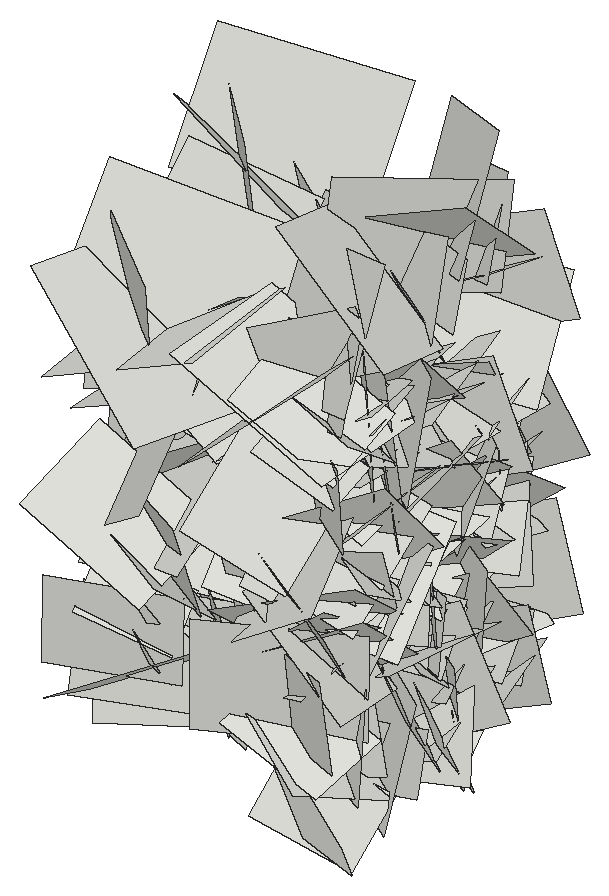
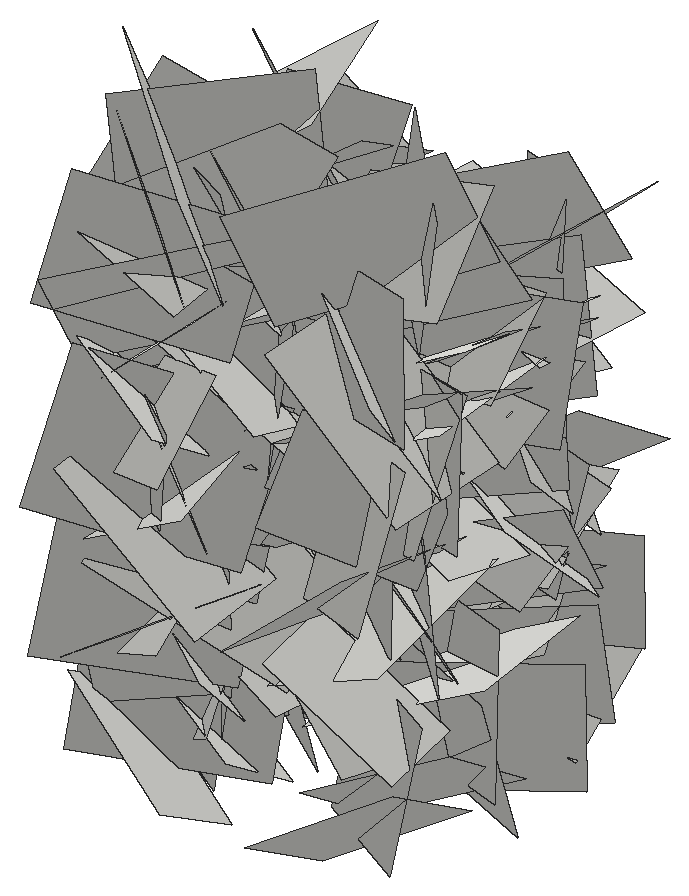
# SketchUp Ruby script. Lengths in inches.
U = 1.inch
M = Sketchup.active_model
def pt(a) = Geom::Point3d.new(a.map { |v| v * U })
def face(e, loops, mat)
  f = e.add_face(loops[0].map { |a| pt(a) })
  loops[1..].each { |l| e.add_face(l.map { |a| pt(a) }).erase! }
  f.material = f.back_material = mat if mat
  f
end
# faces: each face lists its corners as indices into pts; further lists are holes
def faces(e, pts, list, mat = nil) = list.each { |f| face(e, (f[0].is_a?(Array) ? f : [f]).map { |l| l.map { |i| pts[i] } }, mat) }
# xy, xz, yz: faces in a plane at the given z, y or x. An outline is a flat list of corners, or four numbers for a rectangle; further outlines are holes
def ring(l) = l.size == 4 ? [[l[0], l[1]], [l[2], l[1]], [l[2], l[3]], [l[0], l[3]]] : l.each_slice(2).to_a
def flat(e, list, mat, &to3) = list.each { |f| face(e, (f[0].is_a?(Array) ? f : [f]).map { |l| ring(l).map { |u, v| to3.(u, v) } }, mat) }
def xy(e, z, list, mat = nil) = flat(e, list, mat) { |x, y| [x, y, z] }
def xz(e, y, list, mat = nil) = flat(e, list, mat) { |x, z| [x, y, z] }
def yz(e, x, list, mat = nil) = flat(e, list, mat) { |y, z| [x, y, z] }
def lines(e, pts, list) = list.each { |a, b| e.add_line(pt(pts[a]), pt(pts[b])) }
# prism: a flat outline (further loops are holes) pulled along v
def prism(e, loops, v, mat = nil)
  f = face(e, loops, mat); d = Geom::Vector3d.new(v.map { |x| x * U })
  f.pushpull(f.normal.samedirection?(d) ? d.length : -d.length)
end
def box(e, o, s, mat = nil) = prism(e, [[o, [o[0] + s[0], o[1], o[2]], [o[0] + s[0], o[1] + s[1], o[2]], [o[0], o[1] + s[1], o[2]]]], [0, 0, s[2]], mat)
def at(x, y, z, deg = 0) = Geom::Transformation.translation(pt([x, y, z])) * Geom::Transformation.rotation(ORIGIN, Z_AXIS, deg.degrees)
def axes(o, x, y, z) = Geom::Transformation.new([*x, 0, *y, 0, *z, 0, *pt(o).to_a, 1])
def part(name) = M.definitions.add(name)
# library, detail: a bought-in or finely detailed component or shape, given as its bounding box
def library(name, o, s) = part(name).tap { |d| box(d.entities, o, s) }
def detail(e, o, s) = box(e.add_group.entities, o, s)
def put(e, d, t, mat = nil) = e.add_instance(d, t).tap { |i| i.material = mat if mat }
def group(e, t, mat = nil) = e.add_group.tap { |g| g.transformation = t; g.material = mat if mat }.entities
root = M.entities
c1 = part("Component\#6")
p = [[0.01,0,0],[0,3.24,4.54],[4.32,3.24,4.54],[4.33,0,0]]
faces(c1.entities,p,[[0,1,2,3]])
put(root,c1,axes([14.53,158.45,22.43],[-0.19892,0.24365,-1.12098],[0.08242,-1.13056,-0.25875],[1.21318,0.11676,-0.16622]))
put(root,c1,axes([14.53,153.47,7.93],[-0.25077,0.36385,-1.26635],[-0.08689,-1.28818,-0.35481],[1.39394,-0.01484,-0.24993]))
put(root,c1,axes([18.5,151.91,13.09],[0.06029,-0.61389,0.14039],[-0.0496,0.13645,0.61563],[-0.66568,-0.06576,-0.03315]))
put(root,c1,axes([18.5,155.37,8.05],[0.03179,-0.04018,0.69029],[0.07893,0.6871,0.03676],[-0.72868,0.07267,0.03409]))
put(root,c1,axes([18.5,147.25,18.09],[0.11506,-0.20062,0.68841],[0.02156,0.69683,0.19986],[-0.75976,-0.01061,0.10993]))
put(root,c1,axes([18.5,146,16.15],[0.10062,0.63244,0.10884],[-0.07256,0.11937,-0.63396],[-0.67636,0.08128,0.0842]))
put(root,c1,axes([14.53,157.74,11.21],[0.0595,-0.6331,0.72554],[0.06262,0.72766,0.63038],[1.01877,-0.00775,-0.08112]))
put(root,c1,axes([14.53,160.22,19.0625],[-0.13961,-0.68099,-1.03193],[-0.07146,-1.03227,0.68982],[1.30861,-0.12902,-0.07242]))
put(root,c1,axes([18.5,149.02,5.32],[0.19432,-0.67994,0.40742],[0.04988,0.42677,0.69106],[-0.83874,-0.13215,0.13549]))
put(root,c1,axes([14.53,154.9,1.8],[0.03269,0.90387,0.50014],[0.00572,0.50021,-0.90434],[1.09498,-0.0296,-0.01021]))
put(root,c1,axes([18.5,152.72,13.34],[0.14332,-0.62648,-0.12325],[-0.10799,-0.14554,0.62801],[-0.66813,-0.11086,-0.12794]))
put(root,c1,axes([14.53,157.43,12.97],[-0.1074,-0.05602,-1.35571],[-0.22854,-1.34155,0.07155],[1.42001,-0.22014,-0.09102]))
put(root,c1,axes([14.53,151.01,19.39],[0.01021,0.65154,-0.69294],[0.23408,-0.67557,-0.63214],[0.98066,0.15447,0.1581]))
put(root,c1,axes([14.53,148.31,17.26],[0.09379,0.98835,0.28145],[-0.01751,0.28383,-0.99149],[1.08916,-0.08054,-0.04018]))
put(root,c1,axes([14.53,155.4,17.52],[-0.19723,0.3027,-1.19403],[0.0763,-1.20284,-0.31615],[1.30348,0.11621,-0.16216]))
put(root,c1,axes([14.53,145.87,3.84],[0.08046,-0.07863,0.91675],[0.19442,0.90269,0.06223],[0.95574,-0.17701,-0.08983]))
put(root,c1,axes([14.53,148.09,7.11],[-0.15706,0.67864,1.02073],[0.03183,1.02986,-0.68036],[1.29889,0.05683,0.1401]))
put(root,c1,axes([14.53,148.93,-0.125],[-0.17085,0.2332,1.25619],[-0.02467,1.2654,-0.2379],[1.35409,0.05247,0.15416]))
put(root,c1,axes([14.53,158.83,13.98],[0.00743,-1.2386,0.03478],[-0.17851,0.0335,1.22715],[1.30124,0.01167,0.16814]))
put(root,c1,axes([14.53,152.08,1.74],[0.04493,0.85391,0.54577],[0.09586,0.54089,-0.85328],[1.06994,-0.08432,0.05353]))
put(root,c1,axes([14.53,151.75,19.45],[0.16935,0.44212,0.83371],[0.05466,0.84022,-0.45546],[0.99881,-0.12095,-0.11643]))
put(root,c1,axes([18.5,150.18,6.375],[0.17639,-0.58204,-0.33942],[-0.00316,-0.35025,0.59915],[-0.71419,-0.1422,-0.08648]))
put(root,c1,axes([18.5,148.65,3.04],[0.12439,-0.47488,0.46679],[0.05284,0.47892,0.47469],[-0.70386,-0.04797,0.11813]))
put(root,c1,axes([14.53,156.6875,24.44],[0.16473,0.01802,-1.18121],[-0.23771,-1.16927,-0.04735],[1.22945,-0.22849,0.14911]))
put(root,c1,axes([14.53,147.43,1.76],[0.0449,0.15818,1.07958],[0.0304,1.07985,-0.15935],[1.15617,-0.03454,-0.03773]))
put(root,c1,axes([14.53,158.38,15.93],[-0.03304,0.59909,-1.16183],[-0.1621,-1.15585,-0.5919],[1.37611,-0.12177,-0.09762]))
put(root,c1,axes([14.53,156.09,10.89],[0.02844,-1.01096,-0.23497],[0.17327,-0.228,0.99963],[1.08645,0.06282,-0.15327]))
put(root,c1,axes([14.53,159.05,4.5],[0.22831,-0.97739,-0.02602],[-0.01319,-0.02938,1.00067],[1.03632,0.21495,0.01847]))
put(root,c1,axes([14.53,157.5,5.99],[0.02733,0.34478,-1.12821],[-0.04378,-1.12752,-0.34552],[1.24973,-0.04704,0.01257]))
put(root,c1,axes([14.53,147.25,11.15],[0.01251,0.83252,-0.66438],[0.16644,-0.65852,-0.82239],[1.1167,0.08883,0.13002]))
put(root,c1,axes([18.5,155.94,6.59],[0.14653,0.65267,0.04592],[0.0729,0.03218,-0.6644],[-0.6897,0.14207,-0.06047]))
put(root,c1,axes([14.53,153.16,13.74],[0.07693,-1.07175,0.44962],[-0.07215,0.4458,1.07364],[1.22986,0.09319,0.03486]))
put(root,c1,axes([14.53,150.33,13.2],[-0.24126,0.02501,1.36725],[0.05252,1.3853,-0.01709],[1.44858,-0.04606,0.22834]))
put(root,c1,axes([14.53,144.59,11.1],[0.20686,0.83944,0.54314],[0.00436,0.55271,-0.85571],[1.05982,-0.16612,-0.10249]))
put(root,c1,axes([14.53,153.72,24.55],[-0.10736,0.8301,-0.78481],[0.26067,-0.75358,-0.8288],[1.18252,0.24148,0.11144]))
put(root,c1,axes([14.53,148.8125,12.02],[0.02959,0.36254,-1.01381],[0.21176,-0.99828,-0.35148],[1.12146,0.17893,0.09312]))
put(root,c1,axes([14.53,148.37,14.37],[0.13394,0.02599,1.3483],[-0.3112,1.32226,0.00203],[1.39518,0.29244,-0.12899]))
put(root,c1,axes([14.53,151.84,12.71],[0.09641,-0.969,-0.91768],[-0.24854,-0.9171,0.94515],[1.39265,-0.09659,0.2322]))
put(root,c1,axes([14.53,152.41,8.09],[-0.02535,-1.06677,0.60381],[0.0625,0.60222,1.06631],[1.29785,-0.04984,-0.03955]))
put(root,c1,axes([14.53,153.41,21.56],[0.04666,0.60871,1.19242],[-0.17987,1.18598,-0.59916],[1.40769,0.13136,-0.11609]))
put(root,c1,axes([14.53,154.4,5.48],[-0.14525,-0.2612,-1.20099],[0.27145,-1.18798,0.22915],[1.27422,0.2233,-0.18571]))
put(root,c1,axes([14.53,153.21,11.43],[-0.14123,-0.96535,-0.93141],[0.15435,-0.94087,0.95433],[1.41351,0.00629,-0.19727]))
put(root,c1,axes([14.53,157.09,9.16],[0.26081,-0.66319,-0.77037],[0.09697,-0.77495,0.69635],[1.07312,0.23121,0.12431]))
put(root,c1,axes([14.53,149.27,6.59],[-0.15688,1.33929,-0.00269],[0.18956,0.01708,-1.33541],[1.40693,0.14704,0.17962]))
put(root,c1,axes([14.53,149.82,11.51],[0.16938,-0.10345,1.35904],[-0.25816,1.34416,0.13095],[1.4215,0.25644,-0.13816]))
put(root,c1,axes([14.53,155.16,12.125],[0.20792,1.23942,0.0793],[-0.14973,0.10203,-1.24521],[1.30793,-0.18535,-0.15516]))
put(root,c1,axes([14.53,151.77,16.16],[0.14743,1.12249,0.38129],[0.0578,0.37744,-1.13105],[1.25528,-0.14922,0.00729]))
put(root,c1,axes([14.53,145.22,20.96],[0.20751,1.35949,-0.09859],[-0.20583,-0.07077,-1.36145],[1.43011,-0.20745,-0.18164]))
put(root,c1,axes([14.53,149.47,1.18],[0.22795,-1.08393,0.44752],[0.03192,0.45993,1.09954],[1.24263,0.18702,-0.11034]))
put(root,c1,axes([14.53,155.15,17.37],[0.02517,0.60882,-1.16754],[0.2041,-1.15679,-0.59929],[1.38075,0.1599,0.10987]))
put(root,c1,axes([14.53,146.56,18.67],[0.08115,0.67304,1.19325],[0.03541,1.19384,-0.67552],[1.45175,-0.06674,-0.05023]))
put(root,c1,axes([14.53,150.46,17.01],[0.04698,1.34267,-0.16756],[0.13374,-0.17102,-1.33703],[1.42802,-0.02815,0.13073]))
put(root,c1,axes([14.53,150.02,13.53],[0.11354,-0.10924,1.28227],[0.18202,1.27641,0.09439],[1.35193,-0.16268,-0.1204]))
put(root,c1,axes([14.53,153.54,10.59],[0.17173,1.22834,-0.55665],[0.01226,-0.5619,-1.23655],[1.42944,-0.14275,0.07748]))
put(root,c1,axes([14.53,151.36,16.73],[0.05564,-1.33407,-0.12972],[0.26745,-0.11766,1.31218],[1.39538,0.07575,-0.24633]))
put(root,c1,axes([14.53,148.21,18.05],[0.18781,1.38239,0.05917],[0.11095,0.04609,-1.39025],[1.46247,-0.18102,0.09787]))
put(root,c1,axes([28.31,148.21,18.05],[-0.18781,1.38239,0.05917],[-0.11095,0.04609,-1.39025],[-1.46247,-0.18102,0.09787]))
put(root,c1,axes([28.31,151.36,16.73],[-0.05564,-1.33407,-0.12972],[-0.26745,-0.11766,1.31218],[-1.39538,0.07575,-0.24633]))
put(root,c1,axes([28.31,153.54,10.59],[-0.17173,1.22834,-0.55665],[-0.01226,-0.5619,-1.23655],[-1.42944,-0.14275,0.07748]))
put(root,c1,axes([28.31,150.02,13.53],[-0.11354,-0.10924,1.28227],[-0.18202,1.27641,0.09439],[-1.35193,-0.16268,-0.1204]))
put(root,c1,axes([28.31,150.46,17.01],[-0.04698,1.34267,-0.16756],[-0.13374,-0.17102,-1.33703],[-1.42802,-0.02815,0.13073]))
put(root,c1,axes([28.31,146.56,18.67],[-0.08115,0.67304,1.19325],[-0.03541,1.19384,-0.67552],[-1.45175,-0.06674,-0.05023]))
put(root,c1,axes([28.31,155.15,17.37],[-0.02517,0.60882,-1.16754],[-0.2041,-1.15679,-0.59929],[-1.38075,0.1599,0.10987]))
put(root,c1,axes([28.31,149.47,1.18],[-0.22795,-1.08393,0.44752],[-0.03192,0.45993,1.09954],[-1.24263,0.18702,-0.11034]))
put(root,c1,axes([28.31,145.22,20.96],[-0.20751,1.35949,-0.09859],[0.20583,-0.07077,-1.36145],[-1.43011,-0.20745,-0.18164]))
put(root,c1,axes([28.31,151.77,16.16],[-0.14743,1.12249,0.38129],[-0.0578,0.37744,-1.13105],[-1.25528,-0.14922,0.00729]))
put(root,c1,axes([28.31,155.16,12.125],[-0.20792,1.23942,0.0793],[0.14973,0.10203,-1.24521],[-1.30793,-0.18535,-0.15516]))
put(root,c1,axes([28.31,149.82,11.51],[-0.16938,-0.10345,1.35904],[0.25816,1.34416,0.13095],[-1.4215,0.25644,-0.13816]))
put(root,c1,axes([28.31,149.27,6.59],[0.15688,1.33929,-0.00269],[-0.18956,0.01708,-1.33541],[-1.40693,0.14704,0.17962]))
put(root,c1,axes([28.31,157.09,9.16],[-0.26081,-0.66319,-0.77037],[-0.09697,-0.77495,0.69635],[-1.07312,0.23121,0.12431]))
put(root,c1,axes([28.31,153.21,11.43],[0.14123,-0.96535,-0.93141],[-0.15435,-0.94087,0.95433],[-1.41351,0.00629,-0.19727]))
put(root,c1,axes([28.31,148.05,8.79],[-0.07068,0.0827,-1.14811],[-0.1221,-1.14474,-0.07576],[-1.21402,0.11031,0.07447]))
put(root,c1,axes([28.31,154.4,5.48],[0.14525,-0.2612,-1.20099],[-0.27145,-1.18798,0.22915],[-1.27422,0.2233,-0.18571]))
put(root,c1,axes([28.31,153.41,21.56],[-0.04666,0.60871,1.19242],[0.17987,1.18598,-0.59916],[-1.40769,0.13136,-0.11609]))
put(root,c1,axes([28.31,152.41,8.09],[0.02535,-1.06677,0.60381],[-0.0625,0.60222,1.06631],[-1.29785,-0.04984,-0.03955]))
put(root,c1,axes([28.31,151.84,12.71],[-0.09641,-0.969,-0.91768],[0.24854,-0.9171,0.94515],[-1.39265,-0.09659,0.2322]))
put(root,c1,axes([28.31,148.37,14.37],[-0.13394,0.02599,1.3483],[0.3112,1.32226,0.00203],[-1.39518,0.29244,-0.12899]))
put(root,c1,axes([28.31,148.8125,12.02],[-0.02959,0.36254,-1.01381],[-0.21176,-0.99828,-0.35148],[-1.12146,0.17893,0.09312]))
put(root,c1,axes([28.31,153.72,24.55],[0.10736,0.8301,-0.78481],[-0.26067,-0.75358,-0.8288],[-1.18252,0.24148,0.11144]))
put(root,c1,axes([28.31,144.59,11.1],[-0.20686,0.83944,0.54314],[-0.00436,0.55271,-0.85571],[-1.05982,-0.16612,-0.10249]))
put(root,c1,axes([28.31,150.33,13.2],[0.24126,0.02501,1.36725],[-0.05252,1.3853,-0.01709],[-1.44858,-0.04606,0.22834]))
put(root,c1,axes([28.31,153.16,13.74],[-0.07693,-1.07175,0.44962],[0.07215,0.4458,1.07364],[-1.22986,0.09319,0.03486]))
put(root,c1,axes([28.31,147.25,11.15],[-0.01251,0.83252,-0.66438],[-0.16644,-0.65852,-0.82239],[-1.1167,0.08883,0.13002]))
put(root,c1,axes([28.31,157.5,5.99],[-0.02733,0.34478,-1.12821],[0.04378,-1.12752,-0.34552],[-1.24973,-0.04704,0.01257]))
put(root,c1,axes([28.31,159.05,4.5],[-0.22831,-0.97739,-0.02602],[0.01319,-0.02938,1.00067],[-1.03632,0.21495,0.01847]))
put(root,c1,axes([28.31,156.09,10.89],[-0.02844,-1.01096,-0.23497],[-0.17327,-0.228,0.99963],[-1.08645,0.06282,-0.15327]))
put(root,c1,axes([28.31,158.38,15.93],[0.03304,0.59909,-1.16183],[0.1621,-1.15585,-0.5919],[-1.37611,-0.12177,-0.09762]))
put(root,c1,axes([28.31,147.43,1.76],[-0.0449,0.15818,1.07958],[-0.0304,1.07985,-0.15935],[-1.15617,-0.03454,-0.03773]))
put(root,c1,axes([28.31,156.6875,24.44],[-0.16473,0.01802,-1.18121],[0.23771,-1.16927,-0.04735],[-1.22945,-0.22849,0.14911]))
put(root,c1,axes([24.34,148.65,3.04],[-0.12439,-0.47488,0.46679],[-0.05284,0.47892,0.47469],[0.70386,-0.04797,0.11813]))
put(root,c1,axes([24.34,150.18,6.375],[-0.17639,-0.58204,-0.33942],[0.00316,-0.35025,0.59915],[0.71419,-0.1422,-0.08648]))
put(root,c1,axes([28.31,151.75,19.45],[-0.16935,0.44212,0.83371],[-0.05466,0.84022,-0.45546],[-0.99881,-0.12095,-0.11643]))
put(root,c1,axes([28.31,152.08,1.74],[-0.04493,0.85391,0.54577],[-0.09586,0.54089,-0.85328],[-1.06994,-0.08432,0.05353]))
put(root,c1,axes([28.31,158.83,13.98],[-0.00743,-1.2386,0.03478],[0.17851,0.0335,1.22715],[-1.30124,0.01167,0.16814]))
put(root,c1,axes([28.31,148.93,-0.125],[0.17085,0.2332,1.25619],[0.02467,1.2654,-0.2379],[-1.35409,0.05247,0.15416]))
put(root,c1,axes([28.31,148.09,7.11],[0.15706,0.67864,1.02073],[-0.03183,1.02986,-0.68036],[-1.29889,0.05683,0.1401]))
put(root,c1,axes([28.31,145.87,3.84],[-0.08046,-0.07863,0.91675],[-0.19442,0.90269,0.06223],[-0.95574,-0.17701,-0.08983]))
put(root,c1,axes([28.31,155.4,17.52],[0.19723,0.3027,-1.19403],[-0.0763,-1.20284,-0.31615],[-1.30348,0.11621,-0.16216]))
put(root,c1,axes([28.31,148.31,17.26],[-0.09379,0.98835,0.28145],[0.01751,0.28383,-0.99149],[-1.08916,-0.08054,-0.04018]))
put(root,c1,axes([28.31,151.01,19.39],[-0.01021,0.65154,-0.69294],[-0.23408,-0.67557,-0.63214],[-0.98066,0.15447,0.1581]))
put(root,c1,axes([28.31,157.43,12.97],[0.1074,-0.05602,-1.35571],[0.22854,-1.34155,0.07155],[-1.42001,-0.22014,-0.09102]))
put(root,c1,axes([24.34,152.72,13.34],[-0.14332,-0.62648,-0.12325],[0.10799,-0.14554,0.62801],[0.66813,-0.11086,-0.12794]))
put(root,c1,axes([28.31,154.9,1.8],[-0.03269,0.90387,0.50014],[-0.00572,0.50021,-0.90434],[-1.09498,-0.0296,-0.01021]))
put(root,c1,axes([24.34,149.02,5.32],[-0.19432,-0.67994,0.40742],[-0.04988,0.42677,0.69106],[0.83874,-0.13215,0.13549]))
put(root,c1,axes([28.31,160.22,19.0625],[0.13961,-0.68099,-1.03193],[0.07146,-1.03227,0.68982],[-1.30861,-0.12902,-0.07242]))
put(root,c1,axes([28.31,157.74,11.21],[-0.0595,-0.6331,0.72554],[-0.06262,0.72766,0.63038],[-1.01877,-0.00775,-0.08112]))
put(root,c1,axes([24.34,146,16.15],[-0.10062,0.63244,0.10884],[0.07256,0.11937,-0.63396],[0.67636,0.08128,0.0842]))
put(root,c1,axes([24.34,147.25,18.09],[-0.11506,-0.20062,0.68841],[-0.02156,0.69683,0.19986],[0.75976,-0.01061,0.10993]))
put(root,c1,axes([24.34,155.37,8.05],[-0.03179,-0.04018,0.69029],[-0.07893,0.6871,0.03676],[0.72868,0.07267,0.03409]))
put(root,c1,axes([24.34,151.91,13.09],[-0.06029,-0.61389,0.14039],[0.0496,0.13645,0.61563],[0.66568,-0.06576,-0.03315]))
put(root,c1,axes([28.31,153.47,7.93],[0.25077,0.36385,-1.26635],[0.08689,-1.28818,-0.35481],[-1.39394,-0.01484,-0.24993]))
put(root,c1,axes([28.31,158.45,22.43],[0.19892,0.24365,-1.12098],[-0.08242,-1.13056,-0.25875],[-1.21318,0.11676,-0.16622]))
put(root,c1,axes([24.34,151.13,9.12],[-0.15296,0.67587,0.31221],[0.03502,0.32352,-0.68509],[0.78839,0.11676,0.09101]))
put(root,c1,axes([28.31,148.76,4.0625],[-0.10183,-0.75916,-0.2873],[-0.20096,-0.26032,0.75126],[-0.83661,0.15493,-0.14549]))
put(root,c1,axes([28.31,155.05,20.66],[-0.11898,0.43702,0.87755],[0.10329,0.88388,-0.42771],[-1.03402,0.038,-0.1437]))
put(root,c1,axes([28.31,154.79,8.7],[0.06507,0.61236,-0.89404],[0.03144,-0.89608,-0.61173],[-1.14823,0.01016,-0.06741]))
put(root,c1,axes([24.34,151.99,2.12],[-0.1775,0.68354,0.35821],[0.06031,0.37649,-0.69181],[0.81579,0.12089,0.12909]))
put(root,c1,axes([24.34,151.79,4.27],[-0.00282,-0.67031,0.14172],[-0.04158,0.14164,0.66918],[0.72504,0.00552,0.03892]))
put(root,c1,axes([24.34,147.62,1.41],[-0.08717,-0.06025,0.7019],[0.04865,0.70471,0.06586],[0.74517,-0.05306,0.07781]))
put(root,c1,axes([24.34,156.87,7.65],[0.00449,0.50233,-0.39291],[0.02578,-0.39276,-0.50188],[0.67552,0.01165,0.02176]))
put(root,c1,axes([24.34,153.92,20.8125],[0.01755,0.277,-0.54123],[0.05617,-0.54003,-0.27476],[0.64202,0.03967,0.03883]))
put(root,c1,axes([28.31,152.6,3.91],[-0.02426,0.68313,0.69515],[0.0107,0.69547,-0.68312],[-1.03305,-0.00884,-0.0234]))
put(root,c1,axes([24.34,147.13,6.96],[-0.04816,-0.19283,0.63159],[0.07038,0.62854,0.19668],[0.69645,-0.07685,0.0238]))
put(root,c1,axes([28.31,158.68,8.63],[0.07829,-0.94373,0.27717],[-0.10215,0.26967,0.94388],[-1.03759,-0.09775,-0.07202]))
put(root,c1,axes([28.31,152.91,14.99],[0.05042,0.65822,-0.8803],[0.11398,-0.87969,-0.65195],[-1.15954,-0.05785,-0.10236]))
put(root,c1,axes([28.31,159.16,9.85],[0.13765,0.1916,-1.18129],[0.14512,-1.1828,-0.17679],[-1.2602,-0.11528,-0.14939]))
put(root,c1,axes([28.31,157.06,14.03],[0.04606,-0.47436,-0.98882],[0.12961,-0.98133,0.47614],[-1.15527,-0.12901,0.01399]))
put(root,c1,axes([28.31,149.64,15.49],[0.05397,-0.71515,0.49033],[-0.26351,0.45852,0.69456],[-0.88054,-0.18105,-0.1778]))
put(root,c1,axes([24.34,148.39,13.69],[0.056,0.56116,0.2115],[0.06403,0.20626,-0.56234],[0.63244,-0.07057,0.03821]))
put(root,c1,axes([28.31,147.71,9.53],[0.0202,0.73421,-0.62443],[-0.01239,-0.62433,-0.73445],[-1.02159,0.02209,-0.00344]))
put(root,c1,axes([24.34,146.72,8.375],[0.05548,0.31048,0.67068],[-0.12303,0.66747,-0.29994],[0.77368,0.08387,-0.09579]))
put(root,c1,axes([28.31,152.28,1.18],[0.22482,-0.75958,0.923],[0.06114,0.94282,0.76264],[-1.2656,-0.08938,0.2008]))
put(root,c1,axes([28.31,154.73,4.99],[0.23466,-0.21907,1.02966],[-0.17179,1.03255,0.25453],[-1.10257,-0.20751,0.17949]))
put(root,c1,axes([24.34,148.44,10.1],[0.02371,0.59128,0.15103],[0.13632,0.14317,-0.57956],[0.63236,-0.05303,0.11928]))
put(root,c1,axes([24.34,154.81,5.31],[0.03271,-0.68931,-0.29186],[-0.0897,-0.29345,0.68411],[0.78838,-0.00479,0.08995]))
put(root,c1,axes([24.34,155.07,5.6],[-0.26442,-0.95782,0.42161],[-0.12666,0.45666,0.96674],[1.10204,-0.17733,0.21227]))
put(root,c1,axes([28.31,146.38,17.95],[-0.09245,0.38694,0.78979],[0.04684,0.79459,-0.38441],[-0.93107,0.00155,-0.09776]))
put(root,c1,axes([24.34,155.43,2.74],[0.05213,0.12024,0.7107],[-0.06472,0.71048,-0.11598],[0.7613,0.05216,-0.05853]))
put(root,c1,axes([28.31,149.03,14.67],[0.12882,0.64149,-0.81464],[-0.00451,-0.8199,-0.64626],[-1.09909,0.07855,-0.09282]))
put(root,c1,axes([24.34,145.53,10.42],[-0.22479,1.04725,-0.16356],[-0.16331,-0.19548,-1.05191],[1.11161,0.18306,-0.18761]))
put(root,c1,axes([28.31,147.21,13.43],[0.06341,1.09172,0.23851],[0.19798,0.22572,-1.08003],[-1.16785,0.09755,-0.17015]))
put(root,c1,axes([24.34,146.09,12.1875],[-0.18427,0.52878,-0.65011],[0.11203,-0.64482,-0.55274],[0.8812,0.19255,-0.06567]))
put(root,c1,axes([28.31,151.57,3.27],[-0.14157,0.02397,-0.74069],[-0.04702,-0.75154,-0.01632],[-0.78414,0.04073,0.1347]))
put(root,c1,axes([24.34,154.48,3.89],[0.11783,0.23417,0.69133],[-0.11259,0.69704,-0.21902],[0.76547,0.06648,-0.13863]))
put(root,c1,axes([24.34,152.53,7.1875],[0.08757,-0.64703,0.3684],[-0.09594,0.35919,0.65114],[0.78338,0.11632,0.03856]))
put(root,c1,axes([28.31,153.68,-0.24],[-0.08313,-0.05331,0.78078],[-0.05564,0.78328,0.04821],[-0.82769,-0.0473,-0.08166]))
put(root,c1,axes([24.34,155.23,10.47],[-0.04155,0.12694,-0.87349],[-0.11983,-0.86787,-0.12105],[0.92792,-0.10639,-0.05475]))
put(root,c1,axes([28.31,154.93,13.48],[0.13332,0.92748,-0.67904],[0.1887,-0.69057,-0.91025],[-1.20375,-0.00553,-0.2179]))
put(root,c1,axes([28.31,152.46,19.1],[0.24316,-1.11668,0.32256],[0.08367,0.34299,1.13127],[-1.22923,-0.19755,0.14081]))
put(root,c1,axes([28.31,149.625,17.57],[-0.05592,-0.7816,-0.40589],[0.0657,-0.4089,0.77935],[-0.93124,0.01809,0.07936]))
put(root,c1,axes([24.34,153.02,6.56],[0.04835,0.51462,-0.41299],[0.10228,-0.41473,-0.50612],[0.69191,0.02534,0.10368]))
put(root,c1,axes([24.34,155.74,21.65],[-0.00825,-0.17983,-0.66547],[0.14401,-0.65286,0.17483],[0.71636,0.12918,-0.04281]))
put(root,c1,axes([28.31,147.06,-0.97],[-0.01135,-0.66277,0.66685],[0.09721,0.66298,0.66039],[-0.99185,0.07256,0.05709]))
put(root,c1,axes([24.34,154.86,6.54],[-0.11481,0.21277,-0.79232],[0.09254,-0.79167,-0.22453],[0.86468,0.11298,-0.08117]))
put(root,c1,axes([28.31,155.95,10.68],[-0.04823,-0.00518,0.84226],[0.02844,0.84305,0.00663],[-0.89236,0.02715,-0.04531]))
put(root,c1,axes([28.31,146.53,12.92],[-0.03124,-0.05121,0.8385],[0.00373,0.839,0.05136],[-0.89046,0.00531,-0.0292]))
put(root,c1,axes([28.31,152.8,10.75],[0.04843,-0.82009,-0.82841],[0.32646,-0.79109,0.80013],[-1.19171,-0.25004,0.18553]))
put(root,c1,axes([24.34,155.82,10.86],[-0.10869,-0.77244,0.23734],[0.13092,0.22145,0.77409],[0.8465,-0.13343,-0.08925]))
put(root,c1,axes([24.34,156.49,11.61],[-0.16435,-0.92659,-0.48849],[-0.14398,-0.47186,0.93815],[1.10094,-0.20004,0.04977]))
put(root,c1,axes([28.31,153.88,7.81],[-0.12498,-0.19712,-0.75186],[0.05107,-0.76085,0.19192],[-0.82232,-0.01729,0.12619]))
put(root,c1,axes([24.34,154.72,7.86],[0.01434,-0.12328,-0.7123],[0.10241,-0.70572,0.12398],[0.75939,0.0975,-0.00327]))
put(root,c1,axes([28.31,155.22,14.18],[0.0107,0.67836,0.43703],[-0.08223,0.43585,-0.67474],[-0.8514,-0.03357,0.07066]))
put(root,c1,axes([24.34,152.55,8.85],[-0.17208,0.39932,0.93109],[-0.08126,0.93542,-0.41455],[1.07081,0.13515,0.11817]))
put(root,c1,axes([28.31,155.14,21.07],[0.01676,0.7943,-0.14622],[-0.08914,-0.14383,-0.79043],[-0.85145,0.03069,0.07988]))
put(root,c1,axes([24.34,158.76,13.54],[-0.17018,-0.33172,-0.9968],[-0.1229,-0.99662,0.35033],[1.10678,-0.16167,-0.11436]))
put(root,c1,axes([28.31,151.77,10.3],[-0.00621,-0.04081,-0.81439],[-0.02737,-0.814,0.04098],[-0.86391,0.02608,0.00455]))
put(root,c1,axes([28.31,149.67,1.32],[-0.10197,-0.47157,-0.58691],[0.00963,-0.59236,0.47447],[-0.798,0.05311,0.08072]))
put(root,c1,axes([24.34,154.27,5.56],[-0.10843,0.64197,-0.78685],[-0.13439,-0.79271,-0.63027],[1.06801,-0.03458,-0.15919]))
